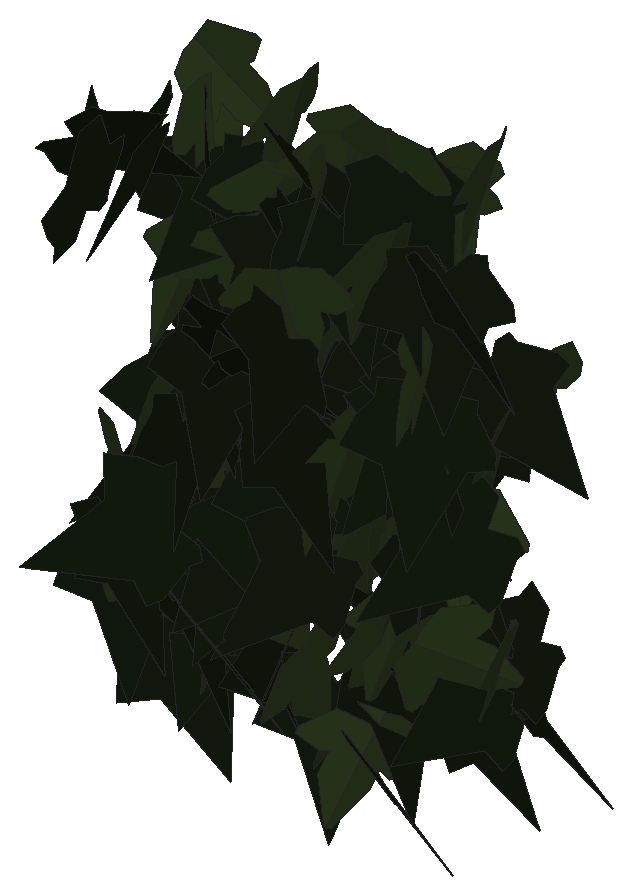
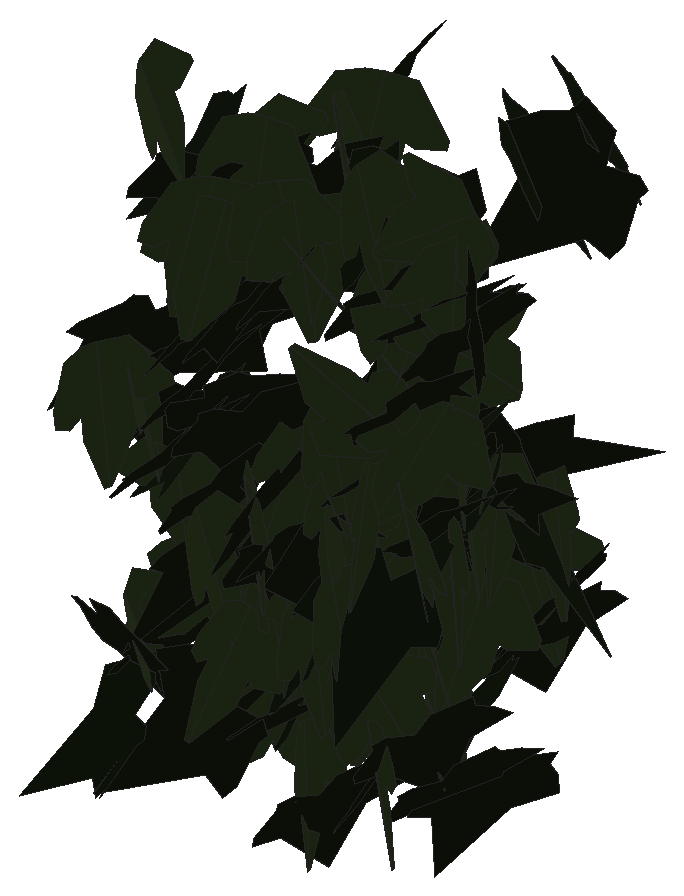
# SketchUp Ruby script. Lengths in inches.
U = 1.inch
M = Sketchup.active_model
def pt(a) = Geom::Point3d.new(a.map { |v| v * U })
def face(e, loops, mat)
  f = e.add_face(loops[0].map { |a| pt(a) })
  loops[1..].each { |l| e.add_face(l.map { |a| pt(a) }).erase! }
  f.material = f.back_material = mat if mat
  f
end
# faces: each face lists its corners as indices into pts; further lists are holes
def faces(e, pts, list, mat = nil) = list.each { |f| face(e, (f[0].is_a?(Array) ? f : [f]).map { |l| l.map { |i| pts[i] } }, mat) }
# xy, xz, yz: faces in a plane at the given z, y or x. An outline is a flat list of corners, or four numbers for a rectangle; further outlines are holes
def ring(l) = l.size == 4 ? [[l[0], l[1]], [l[2], l[1]], [l[2], l[3]], [l[0], l[3]]] : l.each_slice(2).to_a
def flat(e, list, mat, &to3) = list.each { |f| face(e, (f[0].is_a?(Array) ? f : [f]).map { |l| ring(l).map { |u, v| to3.(u, v) } }, mat) }
def xy(e, z, list, mat = nil) = flat(e, list, mat) { |x, y| [x, y, z] }
def xz(e, y, list, mat = nil) = flat(e, list, mat) { |x, z| [x, y, z] }
def yz(e, x, list, mat = nil) = flat(e, list, mat) { |y, z| [x, y, z] }
def lines(e, pts, list) = list.each { |a, b| e.add_line(pt(pts[a]), pt(pts[b])) }
# prism: a flat outline (further loops are holes) pulled along v
def prism(e, loops, v, mat = nil)
  f = face(e, loops, mat); d = Geom::Vector3d.new(v.map { |x| x * U })
  f.pushpull(f.normal.samedirection?(d) ? d.length : -d.length)
end
def box(e, o, s, mat = nil) = prism(e, [[o, [o[0] + s[0], o[1], o[2]], [o[0] + s[0], o[1] + s[1], o[2]], [o[0], o[1] + s[1], o[2]]]], [0, 0, s[2]], mat)
def at(x, y, z, deg = 0) = Geom::Transformation.translation(pt([x, y, z])) * Geom::Transformation.rotation(ORIGIN, Z_AXIS, deg.degrees)
def axes(o, x, y, z) = Geom::Transformation.new([*x, 0, *y, 0, *z, 0, *pt(o).to_a, 1])
def part(name) = M.definitions.add(name)
# library, detail: a bought-in or finely detailed component or shape, given as its bounding box
def library(name, o, s) = part(name).tap { |d| box(d.entities, o, s) }
def detail(e, o, s) = box(e.add_group.entities, o, s)
def put(e, d, t, mat = nil) = e.add_instance(d, t).tap { |i| i.material = mat if mat }
def group(e, t, mat = nil) = e.add_group.tap { |g| g.transformation = t; g.material = mat if mat }.entities
root = M.entities
M.materials.add("efeu1").color = [18, 25, 13]
M.materials.add("efeu2").color = [43, 57, 29]
c1 = part("ivyleaf_9")
p = [[1.54,2.16,1.25],[1.36,2.04,1.19],[-0.21,0.99,0.68],[-0.71,1.11,0.82],[-0.85,0.86,0.67],[-0.8,0.17,0.21],
  [-0.9,-0.01,0.1],[-0.67,-0.16,-0.02],[-0.08,-0.08,-0.05],[-0.03,-0.6,-0.4],[0.65,-0.88,-0.66],[0.83,-0.6,-0.49],
  [1.29,-0.42,-0.43],[1.8125,-0.07,-0.26],[1.21,0.44,0.15]]
faces(c1.entities,p,[[0,1,2,3,4,5,6,7,8,9,10,11,12,13,14]],"efeu1")
c2 = part("ivyleaf_10")
p = [[0,0.5,-0.03],[-0.0625,2.02,-0.43],[-0.19,2.01,-0.46],[-0.54,1.05,-0.29],[-0.52,0.625,-0.18],[-0.83,0.76,-0.28],
  [-1.16,0.64,-0.33],[-1.15,0.33,-0.24],[-0.77,-0.39,0.02],[-0.3,-0.51,0.16],[0.04,-0.48,0.23],[-0.02,2.01,-0.4375],
  [-0.06,2.01,-0.43],[0.04,-0.49,0.23],[0.67,-0.49,0.14],[1.38,0.36,-0.2],[1.375,0.51,-0.24],[0.81,0.65,-0.19],
  [0.62,0.59,-0.15],[0.6,1.09,-0.28],[0.5,1.23,-0.31]]
faces(c2.entities,p,[[0,1,2,3,4,5,6,7,8,9,10],[11,12,0,13,14,15,16,17,18,19,20]],"efeu2")
put(root,c1,axes([34.03,221.97,247.7],[0.02365,-0.11404,-0.48625],[0.49287,-0.07335,0.04117],[-0.08072,-0.48126,0.10894]))
put(root,c1,axes([34.15,220.11,248.22],[0.38628,0.25988,0.18236],[0.15187,0.10096,-0.46556],[-0.2788,0.41506,-0.00094]))
put(root,c2,axes([34.6,220.21,244.83],[-0.37055,0.16154,0.29428],[-0.28168,0.08883,-0.40344],[-0.18262,-0.46477,0.02517]))
put(root,c1,axes([34.65,220.51,244.87],[-0.36922,0.3361,-0.02679],[0.01712,-0.02099,-0.49927],[-0.33673,-0.36959,0.00399]))
put(root,c2,axes([34.48,221.02,245.39],[0.08075,-0.45425,-0.19272],[0.02391,0.19865,-0.45822],[0.49286,0.06479,0.0538]))
put(root,c2,axes([34.53,221.61,245.03],[0.29173,-0.33576,-0.22837],[-0.07126,0.23451,-0.43581],[0.39977,0.28683,0.08897]))
put(root,c2,axes([34.44,221.76,247.99],[0.10521,0.48761,-0.03415],[-0.0443,-0.02528,-0.49739],[-0.48679,0.10768,0.03789]))
put(root,c1,axes([34.4,222.29,243.5],[-0.14251,-0.4788,-0.02105],[0.00459,0.0206,-0.49955],[0.47924,-0.14257,-0.00148]))
put(root,c1,axes([34.37,221.72,247.26],[0.0222,-0.49578,-0.0609],[-0.00545,0.06072,-0.49627],[0.49948,0.02269,-0.00271]))
put(root,c2,axes([34.54,221.27,244.31],[-0.18878,-0.41076,-0.21364],[0.10693,0.18579,-0.45172],[0.45047,-0.21624,0.01769]))
put(root,c2,axes([34.49,222.24,245.5],[0.40118,-0.29098,0.06623],[0.06961,-0.01667,-0.49485],[0.29019,0.40627,0.02714]))
put(root,c1,axes([34.52,221.76,242.78],[-0.17737,-0.46337,0.06189],[0.02468,-0.07538,-0.49367],[0.46683,-0.17207,0.04961]))
put(root,c1,axes([34.47,220.46,243.76],[-0.03932,-0.49616,-0.04774],[-0.00497,0.04827,-0.49764],[0.49843,-0.03866,-0.00873]))
put(root,c1,axes([34.4,220.375,244.03],[0.1712,-0.46464,-0.06931],[-0.00978,0.07023,-0.49495],[0.46968,0.17082,0.01496]))
put(root,c2,axes([34.55,221.3,246.69],[-0.02817,-0.31963,0.38346],[0.16401,-0.36868,-0.29526],[0.47149,0.10915,0.12562]))
put(root,c1,axes([34.89,219.27,248.12],[-0.37105,0.19935,-0.26941],[-0.24553,0.11188,0.42095],[0.22812,0.44468,0.01486]))
put(root,c1,axes([34.69,221.2,245.24],[-0.32717,-0.37765,-0.01848],[0.01249,0.01363,-0.49966],[0.3779,-0.32741,0.00052]))
put(root,c1,axes([34.49,221.19,242.55],[0.00574,-0.43383,-0.24851],[0.04211,0.24807,-0.43208],[0.49819,-0.01597,0.03939]))
put(root,c1,axes([34.78,221.7,245.12],[-0.31416,-0.28136,0.26859],[-0.09474,-0.27951,-0.40361],[0.37727,-0.30448,0.12231]))
put(root,c1,axes([34.72,222.25,246.57],[-0.25914,-0.36981,0.21468],[-0.06095,-0.21652,-0.44655],[0.42324,-0.2576,0.06714]))
put(root,c2,axes([34.77,221.13,245.39],[0.16838,-0.43912,-0.16978],[-0.06167,0.15819,-0.47029],[0.46674,0.17931,-0.00089]))
put(root,c2,axes([34.36,221.79,248.38],[0.26649,0.02972,0.42202],[0.3966,0.15609,-0.26143],[-0.14729,0.47408,0.05962]))
put(root,c2,axes([34.79,220.26,244.22],[-0.09959,-0.47919,0.10225],[-0.0142,-0.10148,-0.48939],[0.48978,-0.10038,0.0066]))
put(root,c2,axes([34.83,222.3,243.21],[0.27657,-0.31752,-0.2696],[-0.13123,0.24072,-0.41813],[0.39533,0.30205,0.04981]))
put(root,c2,axes([34.62,221.81,246.23],[-0.31674,-0.29912,-0.24536],[0.22602,0.11429,-0.43111],[0.31399,-0.38401,0.06281]))
put(root,c1,axes([34.88,220.35,248.43],[-0.38204,0.20798,-0.24655],[0.2115,-0.12703,-0.43489],[-0.24353,-0.43659,0.00909]))
put(root,c1,axes([34.51,221.63,245.14],[0.10783,-0.38061,0.30579],[0.13823,-0.27654,-0.39296],[0.46826,0.16929,0.04559]))
put(root,c1,axes([34.82,222.19,244.78],[0.38934,0.24175,-0.19992],[-0.22927,0.00178,-0.44433],[-0.21412,0.43767,0.11224]))
put(root,c1,axes([34.84,221.72,247.2],[-0.28741,-0.33114,0.2403],[-0.03207,-0.27453,-0.41666],[0.40788,-0.25492,0.13656]))
put(root,c2,axes([34.89,222.34,245.74],[0.12717,-0.42632,-0.2282],[0.02851,0.24216,-0.43651],[0.48272,0.09801,0.0859]))
put(root,c2,axes([34.9,221.51,243.87],[0.34644,-0.35577,0.0584],[0.04449,-0.03819,-0.49655],[0.35778,0.34924,0.00519]))
put(root,c1,axes([34.78,221.5625,245.67],[-0.08219,-0.39898,0.28993],[0.09412,-0.30121,-0.38783],[0.48413,-0.00917,0.12462]))
put(root,c2,axes([34.96,221.3,243.05],[0.21351,-0.44412,0.08471],[0.03606,-0.07666,-0.49277],[0.45068,0.21653,-0.0007]))
put(root,c1,axes([34.7,221.08,243.05],[0.21889,-0.41777,0.16598],[0.0636,-0.15398,-0.47143],[0.44502,0.2275,-0.01427]))
put(root,c2,axes([35.03,222.07,243.59],[-0.19967,-0.38291,0.25202],[0.01828,-0.28132,-0.41295],[0.45804,-0.15569,0.12634]))
put(root,c2,axes([35.09,222.51,244.65],[0.03805,-0.4985,-0.00717],[-0.00068,0.00714,-0.49995],[0.49855,0.03805,-0.00013]))
put(root,c2,axes([35.18,221.3125,244.62],[-0.476,0.09537,0.11971],[-0.12135,0.00316,-0.48504],[-0.09328,-0.49081,0.02014]))
put(root,c2,axes([35.23,221.66,247.37],[-0.08647,-0.41145,0.27062],[-0.0216,-0.27132,-0.41942],[0.49199,-0.08422,0.02915]))
put(root,c2,axes([35.18,221.22,247.01],[-0.33696,-0.33511,-0.15545],[0.13394,0.08526,-0.47412],[0.34427,-0.36116,0.03231]))
put(root,c2,axes([35.27,221.58,245.57],[-0.19216,-0.44184,-0.13362],[0.03966,0.1284,-0.4816],[0.4599,-0.19568,-0.0143]))
put(root,c2,axes([34.96,222.17,246.35],[0.32744,0.11788,-0.359],[0.33863,0.11924,0.34801],[0.16766,-0.47105,-0.00175]))
put(root,c1,axes([35.14,221.78,247.42],[-0.09534,-0.49083,0.00007],[-0.00017,-0.00004,-0.5],[0.49083,-0.09534,-0.00016]))
put(root,c1,axes([35.51,219.72,244.7],[-0.33761,-0.14506,0.33908],[-0.27056,-0.21498,-0.36136],[0.25063,-0.42748,0.06667]))
put(root,c2,axes([35.33,221.83,248.32],[0.04434,-0.49782,0.01453],[0.00207,-0.0144,-0.49979],[0.49803,0.04438,0.00079]))
put(root,c2,axes([35.38,222.08,245.23],[0.11937,-0.48553,-0.00345],[-0.00005,0.00354,-0.49999],[0.48554,0.11936,0.0008]))
put(root,c2,axes([35.4,222.1,245.49],[-0.02635,-0.46498,-0.18192],[0.01079,0.1816,-0.46573],[0.49919,-0.02847,0.00046]))
put(root,c1,axes([35.3,220.19,245.47],[-0.34678,-0.03967,-0.35801],[0.35818,0.01463,-0.34856],[0.03813,-0.49821,0.01827]))
put(root,c2,axes([35.46,222.14,246.15],[-0.00006,-0.49998,0.00418],[-0.00013,-0.00418,-0.49998],[0.5,-0.00006,-0.00013]))
put(root,c1,axes([35.43,221.77,242.34],[-0.16303,-0.17169,0.44039],[-0.07412,-0.4508,-0.20319],[0.46683,-0.13153,0.12154]))
put(root,c2,axes([35.59,221.22,243.46],[-0.19033,-0.42031,-0.19266],[0.07594,0.1771,-0.46138],[0.45608,-0.20489,-0.00358]))
put(root,c1,axes([35.59,220.96,244.08],[-0.24144,-0.35936,0.25014],[-0.02606,-0.27335,-0.41785],[0.43707,-0.21481,0.11326]))
put(root,c1,axes([35.71,220.77,246.17],[-0.12354,0.21997,-0.43168],[0.22696,-0.36732,-0.25213],[-0.42805,-0.25825,-0.00909]))
put(root,c1,axes([35.5,222.46,245.28],[0.08546,-0.48235,-0.10018],[-0.00411,0.10097,-0.48968],[0.49263,0.08452,0.01329]))
put(root,c1,axes([35.68,220.91,244.14],[-0.23953,-0.42361,0.11483],[-0.01568,-0.12247,-0.48451],[0.43861,-0.23571,0.04539]))
put(root,c1,axes([35.53,221.65,244.55],[0.06772,-0.48111,-0.11812],[-0.0035,0.11875,-0.48568],[0.49538,0.06661,0.01271]))
put(root,c1,axes([35.59,220.45,246.23],[-0.04259,-0.48966,0.09176],[-0.00752,-0.09145,-0.49151],[0.49813,-0.04324,0.00042]))
put(root,c1,axes([35.68,222.48,245],[-0.20984,-0.45028,-0.05669],[0.02035,0.05305,-0.49676],[0.45338,-0.21079,-0.00393]))
put(root,c2,axes([35.86,221.99,247.87],[-0.30521,-0.39512,0.02692],[-0.01326,-0.02377,-0.49926],[0.39581,-0.30547,0.00403]))
put(root,c1,axes([36.0625,221.75,247.34],[-0.44642,0.22262,0.03389],[-0.03296,0.00984,-0.49882],[-0.22276,-0.4476,0.00589]))
put(root,c1,axes([35.49,221.52,247.98],[0.42746,-0.25816,0.02524],[0.02318,-0.01045,-0.49935],[0.25835,0.42807,0.00304]))
put(root,c1,axes([35.76,221.31,244.6],[-0.099,-0.4899,-0.01387],[0.00135,0.01388,-0.49981],[0.4901,-0.099,-0.00143]))
put(root,c2,axes([35.91,221.49,244.53],[0.30783,-0.37463,-0.12205],[-0.04049,0.12399,-0.48269],[0.39192,0.30706,0.04599]))
put(root,c2,axes([36.08,222.08,247.99],[-0.45384,-0.09747,0.18583],[-0.1683,-0.0954,-0.46106],[0.12534,-0.48104,0.05379]))
put(root,c2,axes([35.98,221.72,243.83],[-0.06321,-0.49463,-0.03674],[0.00292,0.03666,-0.49865],[0.49598,-0.06325,-0.00175]))
put(root,c1,axes([35.86,221.8,242.17],[-0.09055,-0.48725,-0.06626],[0.00906,0.0657,-0.49558],[0.49165,-0.09095,-0.00307]))
put(root,c1,axes([35.99,221.02,247.12],[-0.25303,-0.35235,0.24865],[-0.01415,-0.28135,-0.41309],[0.43102,-0.21608,0.1324]))
put(root,c1,axes([35.64,220.11,243.43],[0.25809,-0.31414,0.29104],[0.21736,-0.19669,-0.40505],[0.36897,0.3356,0.03504]))
put(root,c2,axes([36.06,222.48,245.29],[0.34073,-0.36479,-0.02872],[0.03276,0.0695,-0.49406],[0.36445,0.33481,0.07126]))
put(root,c1,axes([35.94,222.05,247.45],[0.03872,-0.49559,0.05377],[0.0093,-0.0532,-0.49707],[0.49841,0.03949,0.0051]))
put(root,c1,axes([35.99,222.23,245.46],[0.25971,-0.3379,-0.26149],[-0.131,0.2283,-0.42511],[0.40668,0.28932,0.03006]))
put(root,c1,axes([35.95,221.26,247.17],[0.01768,-0.33179,0.37363],[0.09857,-0.3642,-0.32808],[0.48987,0.08526,0.05254]))
put(root,c1,axes([35.85,219.91,246.83],[0.45391,-0.06054,0.20075],[0.19627,-0.04579,-0.45758],[0.07379,0.4942,-0.01781]))
put(root,c2,axes([36.25,221.47,242.34],[0.13371,-0.45482,-0.15892],[-0.00868,0.16263,-0.47273],[0.48171,0.12918,0.03559]))
put(root,c2,axes([36.23,222.44,243.92],[-0.0869,-0.3633,-0.33235],[0.10327,0.31654,-0.37302],[0.48144,-0.13347,0.02002]))
put(root,c2,axes([36.34,221.64,244.07],[0.00625,-0.47791,-0.14686],[-0.01467,0.14663,-0.47779],[0.49975,0.01029,-0.01219]))
put(root,c2,axes([36.28,221.55,245.33],[-0.09548,-0.39347,-0.29337],[0.09384,0.27872,-0.40436],[0.48175,-0.13227,0.02062]))
put(root,c1,axes([36.02,221.7,243.61],[0.2988,-0.37246,0.1483],[0.08363,-0.12298,-0.47737],[0.39208,0.31008,-0.0112]))
put(root,c1,axes([36.56,220.74,244.29],[-0.48751,-0.10109,0.04597],[-0.04512,-0.00882,-0.49788],[0.10147,-0.4896,-0.00052]))
put(root,c2,axes([36.42,220.81,248.17],[0.24441,-0.40188,-0.16957],[-0.06647,0.15779,-0.46977],[0.4311,0.25218,0.02371]))
put(root,c1,axes([36.43,220.73,243.96],[-0.30483,0.2152,-0.33282],[0.27471,-0.18792,-0.37312],[-0.28567,-0.41034,-0.00367]))
put(root,c1,axes([36.23,220.54,245.68],[0.18338,-0.44648,-0.13049],[-0.04376,0.12308,-0.48264],[0.4631,0.18843,0.00607]))
put(root,c2,axes([36.44,221.11,245.09],[0.02178,-0.4606,0.19332],[0.07408,-0.18838,-0.45719],[0.494,0.04855,0.06003]))
put(root,c2,axes([36.5,222.55,244.85],[0.10123,-0.48804,0.03964],[0.00357,-0.03974,-0.49841],[0.48963,0.10119,-0.00456]))
put(root,c1,axes([36.27,222.31,247.15],[0.10397,-0.48795,-0.03316],[-0.00237,0.0334,-0.49888],[0.48907,0.10389,0.00463]))
put(root,c1,axes([36.43,222.15,245.9],[-0.14726,-0.46226,-0.12097],[0.03001,0.11739,-0.4851],[0.47688,-0.15013,-0.00683]))
put(root,c2,axes([36.63,221.7,248.27],[-0.49732,-0.00574,0.05135],[-0.05144,0.00778,-0.49729],[0.00491,-0.49991,-0.00833]))
put(root,c1,axes([36.61,222.07,242.59],[-0.24537,-0.3401,0.27226],[-0.02821,-0.29941,-0.39944],[0.43474,-0.21138,0.12775]))
put(root,c2,axes([36.65,220.35,243.42],[-0.01395,-0.45143,-0.21452],[0.04845,0.21237,-0.45006],[0.49745,-0.03334,0.03782]))
put(root,c2,axes([36.67,222.24,247.67],[-0.46822,-0.16189,-0.06754],[0.05944,0.03469,-0.49524],[0.16503,-0.47179,-0.01324]))
put(root,c1,axes([36.56,220.97,247.75],[-0.03647,-0.45131,-0.21211],[0.01223,0.2118,-0.45276],[0.49852,-0.03821,-0.00441]))
put(root,c1,axes([36.67,222.27,245.18],[-0.09373,-0.47638,0.11947],[0.00489,-0.12253,-0.48473],[0.49111,-0.0897,0.02763]))
put(root,c2,axes([36.79,222.2,247.84],[-0.28569,-0.38768,-0.13448],[0.12581,0.07322,-0.47834],[0.39058,-0.30716,0.05571]))
put(root,c2,axes([36.95,220.99,242.43],[-0.25746,-0.35655,0.23788],[-0.04016,-0.25621,-0.42749],[0.42673,-0.23923,0.10329]))
put(root,c2,axes([36.92,221.13,243.5],[0.01888,-0.49963,-0.00372],[-0.00072,0.00369,-0.49999],[0.49964,0.01888,-0.00058]))
put(root,c2,axes([36.91,219.73,247.76],[-0.44441,-0.21942,-0.066],[0.05653,0.03457,-0.49559],[0.22204,-0.44795,-0.00592]))
put(root,c1,axes([36.6,222.13,242.93],[0.48651,0.02364,0.11292],[0.11289,0.00336,-0.48708],[-0.02379,0.49943,-0.00207]))
put(root,c2,axes([36.97,221.45,243.62],[-0.04424,-0.44053,0.23232],[0.05939,-0.23624,-0.43665],[0.49448,-0.01104,0.07323]))
put(root,c1,axes([36.78,221.67,248],[0.05207,-0.46366,-0.17974],[0.0378,0.18389,-0.46342],[0.49584,0.03467,0.0542]))
put(root,c2,axes([37.01,221.66,244.08],[0.27823,-0.35802,-0.21074],[0.00533,0.25669,-0.42904],[0.4154,0.2365,0.14665]))
put(root,c1,axes([36.8,221.47,242.79],[0.10696,-0.48798,0.02091],[0.00171,-0.02103,-0.49955],[0.48842,0.10693,-0.00283]))
put(root,c1,axes([37.1875,221.67,245.58],[-0.34049,-0.34468,0.12352],[-0.04025,-0.13241,-0.48046],[0.36393,-0.33713,0.06242]))
put(root,c2,axes([37.2,220.85,247.76],[0.03513,-0.48689,0.10818],[-0.00341,-0.10868,-0.48803],[0.49875,0.03356,-0.01095]))
put(root,c1,axes([37.08,221.61,244.22],[0.15359,-0.31664,-0.35518],[-0.04611,0.36156,-0.34227],[0.47359,0.13789,0.08186]))
put(root,c1,axes([37.17,222.32,245.34],[-0.07798,-0.46713,0.16033],[0.03801,-0.16751,-0.46957],[0.49242,-0.06105,0.06163]))
put(root,c1,axes([37.17,221.8125,246.45],[0.04766,-0.48367,0.11745],[0.03036,-0.11494,-0.48566],[0.4968,0.05342,0.01842]))
put(root,c1,axes([37.14,220.56,242.46],[0.45982,-0.19129,-0.04441],[-0.04096,0.01716,-0.49802],[0.19206,0.46164,0.00011]))
put(root,c1,axes([37.4,221.59,246.04],[-0.21392,-0.43911,0.10685],[-0.03223,-0.10309,-0.48819],[0.45077,-0.21576,0.0158]))
put(root,c1,axes([37.28,219.29,247.48],[-0.02244,-0.43319,0.24868],[0.00576,-0.24914,-0.43347],[0.49946,-0.01659,0.01617]))
put(root,c1,axes([37.19,221.73,245.34],[0.31078,-0.39083,-0.02596],[-0.01008,0.02515,-0.49927],[0.39156,0.31084,0.00775]))
put(root,c1,axes([37.27,221.88,245.77],[0.00905,-0.4834,0.12743],[0.03468,-0.12654,-0.48248],[0.49871,0.01757,0.03124]))
put(root,c1,axes([37.44,221.75,242.65],[0.28386,-0.36353,-0.19305],[-0.08787,0.17558,-0.45984],[0.40212,0.29499,0.03579]))
put(root,c2,axes([37.54,221.62,244.74],[0.48169,0.13007,0.03247],[0.03121,0.00897,-0.49894],[-0.13038,0.4827,0.00053]))
put(root,c1,axes([37.65,221,246.06],[-0.2391,-0.42394,-0.11448],[0.05697,0.0993,-0.48672],[0.43542,-0.24579,0.00081]))
put(root,c2,axes([37.73,221.78,248.52],[0.17265,-0.4611,0.08706],[0.02478,-0.08368,-0.49232],[0.46859,0.17432,-0.00604]))
put(root,c2,axes([37.78,222.43,245.96],[-0.13764,-0.48038,-0.01687],[0.00125,0.01719,-0.4997],[0.48068,-0.1376,-0.00353]))
put(root,c2,axes([37.6,221.1,243.52],[-0.18942,-0.22232,-0.40582],[0.28449,0.28989,-0.2916],[0.36495,-0.34137,0.01668]))
put(root,c2,axes([37.81,220.61,246.86],[0.33256,-0.35898,-0.10264],[-0.06111,0.08327,-0.48922],[0.36833,0.33793,0.0115]))
put(root,c1,axes([37.71,221.12,247.51],[-0.16832,-0.43968,-0.16838],[0.04302,0.16371,-0.47048],[0.46885,-0.17287,-0.01729]))
put(root,c1,axes([37.87,221.67,242.93],[-0.21306,-0.30644,0.33271],[-0.14039,-0.30481,-0.37065],[0.42999,-0.25136,0.04385]))
put(root,c1,axes([38.02,222.08,243.27],[-0.49382,0.05512,-0.05572],[0.05623,0.00151,-0.49683],[-0.0546,-0.49695,-0.00769]))
put(root,c2,axes([37.85,221.81,245.7],[0.20689,-0.45463,-0.02265],[-0.00035,0.02472,-0.49939],[0.45519,0.20665,0.00991]))
put(root,c1,axes([38.1,221.19,244.91],[-0.43891,-0.18733,0.1492],[-0.13918,-0.05397,-0.4772],[0.19489,-0.46043,-0.00476]))
put(root,c1,axes([37.59,222.27,242.5625],[0.43283,-0.25021,-0.00701],[0.01594,0.04153,-0.49802],[0.2498,0.43089,0.04393]))
put(root,c2,axes([37.84,221.84,243.28],[0.2488,-0.40425,0.15709],[0.07646,-0.13738,-0.47464],[0.42691,0.2602,-0.00654]))
put(root,c1,axes([37.7,221.01,247.56],[0.35694,-0.35012,0.00293],[0.00584,0.00178,-0.49996],[0.35009,0.35695,0.00536]))
put(root,c1,axes([37.79,221.72,246.22],[0.10055,-0.33607,-0.35629],[0.06225,0.36954,-0.331],[0.48581,0.0222,0.11616]))
